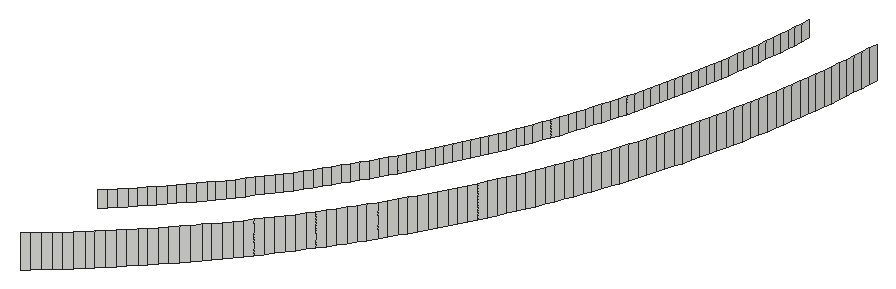
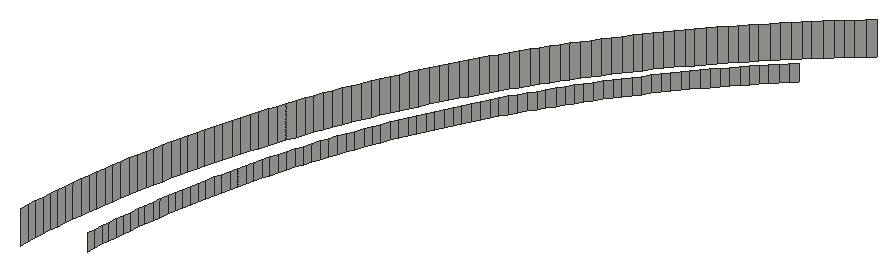
# SketchUp Ruby script. Lengths in inches.
U = 1.inch
M = Sketchup.active_model
def pt(a) = Geom::Point3d.new(a.map { |v| v * U })
def face(e, loops, mat)
  f = e.add_face(loops[0].map { |a| pt(a) })
  loops[1..].each { |l| e.add_face(l.map { |a| pt(a) }).erase! }
  f.material = f.back_material = mat if mat
  f
end
# faces: each face lists its corners as indices into pts; further lists are holes
def faces(e, pts, list, mat = nil) = list.each { |f| face(e, (f[0].is_a?(Array) ? f : [f]).map { |l| l.map { |i| pts[i] } }, mat) }
# xy, xz, yz: faces in a plane at the given z, y or x. An outline is a flat list of corners, or four numbers for a rectangle; further outlines are holes
def ring(l) = l.size == 4 ? [[l[0], l[1]], [l[2], l[1]], [l[2], l[3]], [l[0], l[3]]] : l.each_slice(2).to_a
def flat(e, list, mat, &to3) = list.each { |f| face(e, (f[0].is_a?(Array) ? f : [f]).map { |l| ring(l).map { |u, v| to3.(u, v) } }, mat) }
def xy(e, z, list, mat = nil) = flat(e, list, mat) { |x, y| [x, y, z] }
def xz(e, y, list, mat = nil) = flat(e, list, mat) { |x, z| [x, y, z] }
def yz(e, x, list, mat = nil) = flat(e, list, mat) { |y, z| [x, y, z] }
def lines(e, pts, list) = list.each { |a, b| e.add_line(pt(pts[a]), pt(pts[b])) }
# prism: a flat outline (further loops are holes) pulled along v
def prism(e, loops, v, mat = nil)
  f = face(e, loops, mat); d = Geom::Vector3d.new(v.map { |x| x * U })
  f.pushpull(f.normal.samedirection?(d) ? d.length : -d.length)
end
def box(e, o, s, mat = nil) = prism(e, [[o, [o[0] + s[0], o[1], o[2]], [o[0] + s[0], o[1] + s[1], o[2]], [o[0], o[1] + s[1], o[2]]]], [0, 0, s[2]], mat)
def at(x, y, z, deg = 0) = Geom::Transformation.translation(pt([x, y, z])) * Geom::Transformation.rotation(ORIGIN, Z_AXIS, deg.degrees)
def axes(o, x, y, z) = Geom::Transformation.new([*x, 0, *y, 0, *z, 0, *pt(o).to_a, 1])
def part(name) = M.definitions.add(name)
# library, detail: a bought-in or finely detailed component or shape, given as its bounding box
def library(name, o, s) = part(name).tap { |d| box(d.entities, o, s) }
def detail(e, o, s) = box(e.add_group.entities, o, s)
def put(e, d, t, mat = nil) = e.add_instance(d, t).tap { |i| i.material = mat if mat }
def group(e, t, mat = nil) = e.add_group.tap { |g| g.transformation = t; g.material = mat if mat }.entities
root = M.entities
p = [[336.86,165.46,107.5],[336.66,165.3,107.5],[336.66,165.3,108.5],[336.86,165.46,108.5],[337.05,165.63,107.5],[337.05,165.63,108.5],
  [337.24,165.8,107.5],[337.24,165.8,108.5],[337.4375,165.97,107.5],[337.4375,165.97,108.5],[337.625,166.14,107.5],[337.625,166.14,108.5],
  [337.8125,166.32,107.5],[337.8125,166.32,108.5],[338,166.49,107.5],[338,166.49,108.5],[338.1875,166.67,107.5],[338.1875,166.67,108.5],
  [338.37,166.85,107.5],[338.37,166.85,108.5],[338.55,167.03,107.5],[338.55,167.03,108.5],[338.73,167.22,107.5],[338.73,167.22,108.5],
  [338.91,167.4,107.5],[338.91,167.4,108.5],[339.09,167.59,107.5],[339.09,167.59,108.5],[339.26,167.77,107.5],[339.26,167.77,108.5],
  [339.4375,167.96,107.5],[339.4375,167.96,108.5],[339.61,168.15,107.5],[339.61,168.15,108.5],[339.78,168.35,107.5],[339.78,168.35,108.5],
  [339.95,168.54,107.5],[339.95,168.54,108.5],[340.12,168.74,107.5],[340.12,168.74,108.5],[340.28,168.93,107.5],[340.28,168.93,108.5],
  [340.45,169.13,107.5],[340.45,169.13,108.5],[340.61,169.33,107.5],[340.61,169.33,108.5],[340.77,169.53,107.5],[340.77,169.53,108.5],
  [340.93,169.73,107.5],[340.93,169.73,108.5],[341.08,169.9375,107.5],[341.08,169.9375,108.5],[341.24,170.14,107.5],[341.24,170.14,108.5],
  [341.39,170.35,107.5],[341.39,170.35,108.5],[341.54,170.56,107.5],[341.54,170.56,108.5],[341.69,170.77,107.5],[341.69,170.77,108.5],
  [341.84,170.98,107.5],[341.84,170.98,108.5],[341.98,171.1875,107.5],[341.98,171.1875,108.5],[342.125,171.4,107.5],[342.125,171.4,108.5],
  [342.27,171.61,107.5],[342.27,171.61,108.5],[342.41,171.83,107.5],[342.41,171.83,108.5],[342.55,172.05,107.5],[342.55,172.05,108.5],
  [342.68,172.27,107.5],[342.68,172.27,108.5],[342.82,172.48,107.5],[342.82,172.48,108.5],[342.95,172.7,107.5],[342.95,172.7,108.5],
  [343.08,172.93,107.5],[343.08,172.93,108.5],[343.21,173.15,107.5],[343.21,173.15,108.5],[343.33,173.37,107.5],[343.33,173.37,108.5],
  [343.46,173.6,107.5],[343.46,173.6,108.5],[343.58,173.82,107.5],[343.58,173.82,108.5],[343.7,174.05,107.5],[343.7,174.05,108.5],
  [343.82,174.28,107.5],[343.82,174.28,108.5],[343.93,174.51,107.5],[343.93,174.51,108.5],[344.05,174.74,107.5],[344.05,174.74,108.5],
  [344.16,174.97,107.5],[344.16,174.97,108.5],[344.27,175.2,107.5],[344.27,175.2,108.5],[344.375,175.43,107.5],[344.375,175.43,108.5],
  [344.48,175.67,107.5],[344.48,175.67,108.5],[344.59,175.9,107.5],[344.59,175.9,108.5],[344.6875,176.14,107.5],[344.6875,176.14,108.5],
  [344.79,176.375,107.5],[344.79,176.375,108.5],[344.88,176.61,107.5],[344.88,176.61,108.5],[344.98,176.85,107.5],[344.98,176.85,108.5],
  [345.07,177.09,107.5],[345.07,177.09,108.5],[345.16,177.33,107.5],[345.16,177.33,108.5],[345.25,177.57,107.5],[345.25,177.57,108.5],
  [345.34,177.82,107.5],[345.34,177.82,108.5],[345.42,178.06,107.5],[345.42,178.06,108.5],[345.51,178.3,107.5],[345.51,178.3,108.5],
  [345.59,178.55,107.5],[345.59,178.55,108.5],[345.67,178.79,107.5],[345.67,178.79,108.5],[345.74,179.04,107.5],[345.74,179.04,108.5],
  [345.82,179.28,107.5],[345.82,179.28,108.5],[345.89,179.53,107.5],[345.89,179.53,108.5],[345.96,179.78,107.5],[345.96,179.78,108.5],
  [346.02,180.02,107.5],[346.02,180.02,108.5],[346.09,180.27,107.5],[346.09,180.27,108.5],[346.15,180.52,107.5],[346.15,180.52,108.5],
  [346.21,180.77,107.5],[346.21,180.77,108.5],[346.27,181.02,107.5],[346.27,181.02,108.5],[346.33,181.27,107.5],[346.33,181.27,108.5],
  [346.38,181.52,107.5],[346.38,181.52,108.5],[346.43,181.77,107.5],[346.43,181.77,108.5],[346.48,182.03,107.5],[346.48,182.03,108.5],
  [346.53,182.28,107.5],[346.53,182.28,108.5],[346.58,182.53,107.5],[346.58,182.53,108.5],[346.62,182.79,107.5],[346.62,182.79,108.5],
  [346.66,183.04,107.5],[346.66,183.04,108.5],[346.7,183.29,107.5],[346.7,183.29,108.5],[346.73,183.55,107.5],[346.73,183.55,108.5],
  [346.77,183.8,107.5],[346.77,183.8,108.5],[346.8,184.06,107.5],[346.8,184.06,108.5],[346.83,184.3125,107.5],[346.83,184.3125,108.5],
  [346.86,184.57,107.5],[346.86,184.57,108.5],[346.88,184.82,107.5],[346.88,184.82,108.5],[346.9,185.08,107.5],[346.9,185.08,108.5],
  [346.92,185.34,107.5],[346.92,185.34,108.5],[336.79,168.11,108],[336.97,168.28,108],[336.97,168.28,108.5],[336.79,168.11,108.5],
  [337.13,168.44,108],[337.13,168.44,108.5],[337.3,168.62,108],[337.3,168.62,108.5],[337.47,168.79,108],[337.47,168.79,108.5],
  [337.63,168.96,108],[337.63,168.96,108.5],[337.8,169.13,108],[337.8,169.13,108.5],[337.96,169.3125,108],[337.96,169.3125,108.5],
  [338.12,169.49,108],[338.12,169.49,108.5],[338.28,169.67,108],[338.28,169.67,108.5],[338.4375,169.85,108],[338.4375,169.85,108.5],
  [338.59,170.03,108],[338.59,170.03,108.5],[338.75,170.21,108],[338.75,170.21,108.5],[338.9,170.4,108],[338.9,170.4,108.5],
  [339.05,170.58,108],[339.05,170.58,108.5],[339.2,170.77,108],[339.2,170.77,108.5],[339.34,170.96,108],[339.34,170.96,108.5],
  [339.49,171.15,108],[339.49,171.15,108.5],[339.63,171.34,108],[339.63,171.34,108.5],[339.78,171.53,108],[339.78,171.53,108.5],
  [339.92,171.72,108],[339.92,171.72,108.5],[340.06,171.92,108],[340.06,171.92,108.5],[340.19,172.12,108],[340.19,172.12,108.5],
  [340.33,172.3125,108],[340.33,172.3125,108.5],[340.46,172.51,108],[340.46,172.51,108.5],[340.59,172.71,108],[340.59,172.71,108.5],
  [340.72,172.91,108],[340.72,172.91,108.5],[340.85,173.11,108],[340.85,173.11,108.5],[340.98,173.32,108],[340.98,173.32,108.5],
  [341.1,173.52,108],[341.1,173.52,108.5],[341.23,173.72,108],[341.23,173.72,108.5],[341.35,173.93,108],[341.35,173.93,108.5],
  [341.47,174.14,108],[341.47,174.14,108.5],[341.58,174.35,108],[341.58,174.35,108.5],[341.7,174.56,108],[341.7,174.56,108.5],
  [341.8125,174.77,108],[341.8125,174.77,108.5],[341.93,174.98,108],[341.93,174.98,108.5],[342.04,175.19,108],[342.04,175.19,108.5],
  [342.14,175.4,108],[342.14,175.4,108.5],[342.25,175.62,108],[342.25,175.62,108.5],[342.35,175.83,108],[342.35,175.83,108.5],
  [342.46,176.05,108],[342.46,176.05,108.5],[342.56,176.27,108],[342.56,176.27,108.5],[342.66,176.48,108],[342.66,176.48,108.5],
  [342.75,176.7,108],[342.75,176.7,108.5],[342.85,176.92,108],[342.85,176.92,108.5],[342.94,177.14,108],[342.94,177.14,108.5],
  [343.03,177.37,108],[343.03,177.37,108.5],[343.12,177.59,108],[343.12,177.59,108.5],[343.21,177.81,108],[343.21,177.81,108.5],
  [343.29,178.03,108],[343.29,178.03,108.5],[343.375,178.26,108],[343.375,178.26,108.5],[343.45,178.48,108],[343.45,178.48,108.5],
  [343.53,178.71,108],[343.53,178.71,108.5],[343.61,178.9375,108],[343.61,178.9375,108.5],[343.68,179.16,108],[343.68,179.16,108.5],
  [343.76,179.39,108],[343.76,179.39,108.5],[343.83,179.62,108],[343.83,179.62,108.5],[343.9,179.85,108],[343.9,179.85,108.5],
  [343.96,180.08,108],[343.96,180.08,108.5],[344.03,180.31,108],[344.03,180.31,108.5],[344.09,180.54,108],[344.09,180.54,108.5],
  [344.15,180.77,108],[344.15,180.77,108.5],[344.21,181,108],[344.21,181,108.5],[344.27,181.23,108],[344.27,181.23,108.5],
  [344.32,181.47,108],[344.32,181.47,108.5],[344.375,181.7,108],[344.375,181.7,108.5],[344.42,181.93,108],[344.42,181.93,108.5],
  [344.47,182.17,108],[344.47,182.17,108.5],[344.52,182.4,108],[344.52,182.4,108.5],[344.5625,182.64,108],[344.5625,182.64,108.5],
  [344.6,182.875,108],[344.6,182.875,108.5],[344.64,183.11,108],[344.64,183.11,108.5],[344.68,183.35,108],[344.68,183.35,108.5],
  [344.72,183.58,108],[344.72,183.58,108.5],[344.75,183.82,108],[344.75,183.82,108.5],[344.78,184.06,108],[344.78,184.06,108.5],
  [344.8125,184.29,108],[344.8125,184.29,108.5],[344.84,184.53,108],[344.84,184.53,108.5],[344.87,184.77,108],[344.87,184.77,108.5],
  [344.89,185.01,108],[344.89,185.01,108.5],[344.91,185.25,108],[344.91,185.25,108.5]]
faces(root,p,[[0,1,2,3],[4,0,3,5],[6,4,5,7],[8,6,7,9],[10,8,9,11],[12,10,11,13],[14,12,13,15],[16,14,15,17],
  [18,16,17,19],[20,18,19,21],[22,20,21,23],[24,22,23,25],[26,24,25,27],[28,26,27,29],[30,28,29,31],[32,30,31,33],
  [34,32,33,35],[36,34,35,37],[38,36,37,39],[40,38,39,41],[42,40,41,43],[44,42,43,45],[46,44,45,47],[48,46,47,49],
  [50,48,49,51],[52,50,51,53],[54,52,53,55],[56,54,55,57],[58,56,57,59],[60,58,59,61],[62,60,61,63],[64,62,63,65],
  [66,64,65,67],[68,66,67,69],[70,68,69,71],[72,70,71,73],[74,72,73,75],[76,74,75,77],[78,76,77,79],[80,78,79,81],
  [82,80,81,83],[84,82,83,85],[86,84,85,87],[88,86,87,89],[90,88,89,91],[92,90,91,93],[94,92,93,95],[96,94,95,97],
  [98,96,97,99],[100,98,99,101],[102,100,101,103],[104,102,103,105],[106,104,105,107],[108,106,107,109],[110,108,109,111],[112,110,111,113],
  [114,112,113,115],[116,114,115,117],[118,116,117,119],[120,118,119,121],[122,120,121,123],[124,122,123,125],[126,124,125,127],[128,126,127,129],
  [130,128,129,131],[132,130,131,133],[134,132,133,135],[136,134,135,137],[138,136,137,139],[140,138,139,141],[142,140,141,143],[144,142,143,145],
  [146,144,145,147],[148,146,147,149],[150,148,149,151],[152,150,151,153],[154,152,153,155],[156,154,155,157],[158,156,157,159],[160,158,159,161],
  [162,160,161,163],[164,162,163,165],[166,164,165,167],[168,166,167,169],[170,168,169,171],[172,170,171,173],[174,172,173,175],[176,174,175,177],
  [178,176,177,179],[180,178,179,181],[182,183,184,185],[183,186,187,184],[186,188,189,187],[188,190,191,189],[190,192,193,191],[192,194,195,193],
  [194,196,197,195],[196,198,199,197],[198,200,201,199],[200,202,203,201],[202,204,205,203],[204,206,207,205],[206,208,209,207],[208,210,211,209],
  [210,212,213,211],[212,214,215,213],[214,216,217,215],[216,218,219,217],[218,220,221,219],[220,222,223,221],[222,224,225,223],[224,226,227,225],
  [226,228,229,227],[228,230,231,229],[230,232,233,231],[232,234,235,233],[234,236,237,235],[236,238,239,237],[238,240,241,239],[240,242,243,241],
  [242,244,245,243],[244,246,247,245],[246,248,249,247],[248,250,251,249],[250,252,253,251],[252,254,255,253],[254,256,257,255],[256,258,259,257],
  [258,260,261,259],[260,262,263,261],[262,264,265,263],[264,266,267,265],[266,268,269,267],[268,270,271,269],[270,272,273,271],[272,274,275,273],
  [274,276,277,275],[276,278,279,277],[278,280,281,279],[280,282,283,281],[282,284,285,283],[284,286,287,285],[286,288,289,287],[288,290,291,289],
  [290,292,293,291],[292,294,295,293],[294,296,297,295],[296,298,299,297],[298,300,301,299],[300,302,303,301],[302,304,305,303],[304,306,307,305],
  [306,308,309,307],[308,310,311,309],[310,312,313,311],[312,314,315,313],[314,316,317,315],[316,318,319,317],[318,320,321,319],[320,322,323,321],
  [322,324,325,323],[324,326,327,325],[326,328,329,327],[328,330,331,329],[330,332,333,331],[332,334,335,333],[334,336,337,335],[336,338,339,337],
  [338,340,341,339],[340,342,343,341],[342,344,345,343]])
